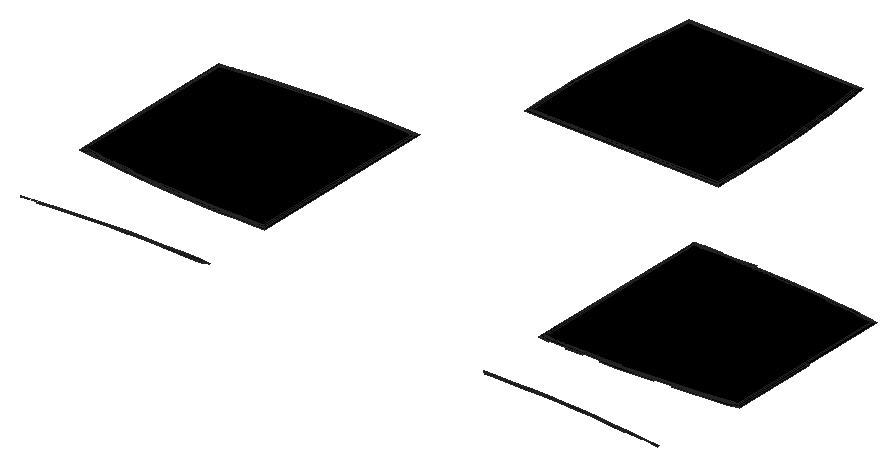
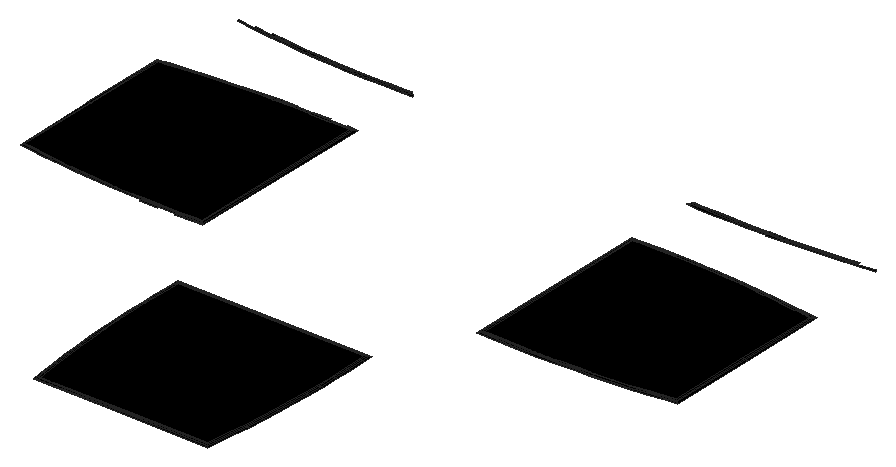
# SketchUp Ruby script. Lengths in inches.
U = 1.inch
M = Sketchup.active_model
def pt(a) = Geom::Point3d.new(a.map { |v| v * U })
def face(e, loops, mat)
  f = e.add_face(loops[0].map { |a| pt(a) })
  loops[1..].each { |l| e.add_face(l.map { |a| pt(a) }).erase! }
  f.material = f.back_material = mat if mat
  f
end
# faces: each face lists its corners as indices into pts; further lists are holes
def faces(e, pts, list, mat = nil) = list.each { |f| face(e, (f[0].is_a?(Array) ? f : [f]).map { |l| l.map { |i| pts[i] } }, mat) }
# xy, xz, yz: faces in a plane at the given z, y or x. An outline is a flat list of corners, or four numbers for a rectangle; further outlines are holes
def ring(l) = l.size == 4 ? [[l[0], l[1]], [l[2], l[1]], [l[2], l[3]], [l[0], l[3]]] : l.each_slice(2).to_a
def flat(e, list, mat, &to3) = list.each { |f| face(e, (f[0].is_a?(Array) ? f : [f]).map { |l| ring(l).map { |u, v| to3.(u, v) } }, mat) }
def xy(e, z, list, mat = nil) = flat(e, list, mat) { |x, y| [x, y, z] }
def xz(e, y, list, mat = nil) = flat(e, list, mat) { |x, z| [x, y, z] }
def yz(e, x, list, mat = nil) = flat(e, list, mat) { |y, z| [x, y, z] }
def lines(e, pts, list) = list.each { |a, b| e.add_line(pt(pts[a]), pt(pts[b])) }
# prism: a flat outline (further loops are holes) pulled along v
def prism(e, loops, v, mat = nil)
  f = face(e, loops, mat); d = Geom::Vector3d.new(v.map { |x| x * U })
  f.pushpull(f.normal.samedirection?(d) ? d.length : -d.length)
end
def box(e, o, s, mat = nil) = prism(e, [[o, [o[0] + s[0], o[1], o[2]], [o[0] + s[0], o[1] + s[1], o[2]], [o[0], o[1] + s[1], o[2]]]], [0, 0, s[2]], mat)
def at(x, y, z, deg = 0) = Geom::Transformation.translation(pt([x, y, z])) * Geom::Transformation.rotation(ORIGIN, Z_AXIS, deg.degrees)
def axes(o, x, y, z) = Geom::Transformation.new([*x, 0, *y, 0, *z, 0, *pt(o).to_a, 1])
def part(name) = M.definitions.add(name)
# library, detail: a bought-in or finely detailed component or shape, given as its bounding box
def library(name, o, s) = part(name).tap { |d| box(d.entities, o, s) }
def detail(e, o, s) = box(e.add_group.entities, o, s)
def put(e, d, t, mat = nil) = e.add_instance(d, t).tap { |i| i.material = mat if mat }
def group(e, t, mat = nil) = e.add_group.tap { |g| g.transformation = t; g.material = mat if mat }.entities
root = M.entities
M.materials.add("[Color M09]").color = [0, 0, 0]
xy(root,29.97,[[96.41,139.98,98.1,140,99.78,140.04,100.4,140.0625,100.4,158.33,99.78,158.35,98.1,158.39,96.41,158.41,94.72,158.39,93.04,158.35,93.02,158.35,91.35,158.28,89.66,158.18,87.98,158.06,86.3,157.9,84.62,157.72,82.94,157.51,82.23,157.41,82.23,140.98,82.94,140.88,84.62,140.67,86.3,140.49,87.98,140.33,89.66,140.21,91.35,140.11,93.02,140.04,93.04,140.04,94.72,140],[132.31,139.98,134,140,135.68,140.04,135.7,140.04,137.375,140.11,139.0625,140.21,140.75,140.33,142.43,140.49,144.1,140.67,145.78,140.88,146.49,140.98,146.49,157.41,145.78,157.51,144.1,157.72,142.43,157.9,140.75,158.06,139.0625,158.18,137.375,158.28,135.7,158.35,135.68,158.35,134,158.39,132.31,158.41,130.625,158.39,128.9375,158.35,128.32,158.33,128.32,140.0625,128.9375,140.04,130.625,140],[105.23,167.19,123.49,167.19,123.52,167.8125,123.56,169.5,123.57,171.1875,123.56,172.875,123.52,174.55,123.52,174.57,123.45,176.25,123.35,177.93,123.22,179.62,123.07,181.3,122.89,182.98,122.68,184.65,122.58,185.37,106.15,185.37,106.05,184.65,105.84,182.98,105.65,181.3,105.5,179.62,105.375,177.93,105.28,176.25,105.21,174.57,105.21,174.55,105.16,172.875,105.15,171.1875,105.16,169.5,105.21,167.8125]],"[Color M09]")
p = [[84.59,132.1,29.93],[84.57,132.24,29.89],[82.89,132.03,29.89],[82.91,131.89,29.93],[144.15,132.24,29.89],[144.14,132.1,29.93],
  [145.82,131.89,29.93],[145.84,132.03,29.89],[86.28,132.14,29.96],[86.27,132.28,29.93],[84.6,131.96,29.96],[142.46,132.28,29.93],
  [142.44,132.14,29.96],[144.12,131.96,29.96],[86.25,132.42,29.89],[87.97,132.3,29.96],[87.95,132.44,29.93],[140.77,132.44,29.93],
  [140.76,132.3,29.96],[142.47,132.42,29.89],[87.94,132.58,29.89],[89.65,132.42,29.96],[89.64,132.57,29.93],[139.08,132.57,29.93],
  [139.07,132.42,29.96],[140.78,132.58,29.89],[89.63,132.71,29.89],[91.34,132.52,29.96],[91.33,132.66,29.93],[137.39,132.66,29.93],
  [137.38,132.52,29.96],[139.09,132.71,29.89],[93.02,132.74,29.93],[93.02,132.59,29.96],[135.71,132.74,29.93],[135.7,132.59,29.96],
  [91.33,132.8,29.89],[93.04,132.59,29.96],[93.03,132.74,29.93],[94.72,132.78,29.93],[94.72,132.63,29.96],[96.41,132.79,29.93],
  [96.41,132.65,29.96],[98.1,132.78,29.93],[98.1,132.63,29.96],[99.79,132.74,29.93],[99.79,132.59,29.96],[100.69,132.7,29.93],
  [100.55,132.56,29.96],[128.93,132.74,29.93],[128.93,132.59,29.96],[128.18,132.56,29.96],[128.03,132.7,29.93],[130.62,132.78,29.93],
  [130.625,132.63,29.96],[132.31,132.79,29.93],[132.31,132.65,29.96],[134.01,132.78,29.93],[134.01,132.63,29.96],[135.69,132.74,29.93],
  [135.6875,132.59,29.96],[137.4,132.8,29.89],[93.01,132.875,29.89],[93.02,132.875,29.89],[94.71,132.92,29.89],[98.1,132.92,29.89],
  [99.8,132.875,29.89],[100.83,132.83,29.89],[128.92,132.875,29.89],[127.89,132.83,29.89],[130.62,132.92,29.89],[134.01,132.92,29.89],
  [135.7,132.875,29.89],[135.71,132.875,29.89],[96.41,132.93,29.89],[132.31,132.93,29.89],[91.33,139.68,29.89],[93.01,139.61,29.89],
  [93.02,139.75,29.93],[91.33,139.82,29.93],[94.71,139.57,29.89],[93.02,139.61,29.89],[93.03,139.75,29.93],[94.72,139.7,29.93],
  [96.41,139.69,29.93],[96.41,139.55,29.89],[98.1,139.7,29.93],[98.1,139.56,29.89],[99.79,139.75,29.93],[99.8,139.61,29.89],
  [100.69,139.78,29.93],[100.83,139.65,29.89],[100.69,158.6,29.93],[100.83,158.74,29.89],[128.93,139.75,29.93],[128.92,139.61,29.89],
  [127.89,139.65,29.89],[128.03,139.78,29.93],[127.89,158.74,29.89],[128.03,158.6,29.93],[132.31,139.69,29.93],[132.31,139.55,29.89],
  [130.62,139.56,29.89],[130.62,139.7,29.93],[135.7,139.61,29.89],[134.01,139.57,29.89],[134.01,139.7,29.93],[135.69,139.75,29.93],
  [135.71,139.61,29.89],[137.4,139.68,29.89],[137.39,139.82,29.93],[135.71,139.75,29.93],[89.64,139.92,29.93],[89.63,139.78,29.89],
  [93.02,139.89,29.96],[91.34,139.96,29.96],[93.04,139.89,29.96],[94.72,139.85,29.96],[96.41,139.83,29.96],[98.1,139.85,29.96],
  [99.79,139.89,29.96],[100.55,139.92,29.96],[128.93,139.89,29.96],[128.18,139.92,29.96],[130.625,139.85,29.96],[132.31,139.83,29.96],
  [134.01,139.85,29.96],[135.6875,139.89,29.96],[135.7,139.89,29.96],[137.38,139.96,29.96],[139.09,139.78,29.89],[139.08,139.92,29.93],
  [87.95,140.04,29.93],[87.94,139.9,29.89],[89.65,140.06,29.96],[100.55,158.47,29.96],[128.18,158.47,29.96],[139.07,140.06,29.96],
  [86.27,140.2,29.93],[86.25,140.06,29.89],[87.97,140.1875,29.96],[140.77,140.04,29.93],[140.76,140.1875,29.96],[140.78,139.9,29.89],
  [142.47,140.06,29.89],[142.46,140.2,29.93],[86.28,140.34,29.96],[142.44,140.34,29.96],[84.59,140.38,29.93],[84.57,140.24,29.89],
  [144.15,140.24,29.89],[144.14,140.38,29.93],[82.91,140.59,29.93],[82.89,140.45,29.89],[84.6,140.52,29.96],[144.12,140.52,29.96],
  [145.84,140.45,29.89],[145.82,140.59,29.93],[82.92,140.73,29.96],[145.8,140.73,29.96],[81.9375,140.73,29.93],[81.8,140.61,29.89],
  [146.92,140.61,29.89],[146.78,140.73,29.93],[81.9375,149.19,29.93],[81.8,149.19,29.89],[82.08,140.85,29.96],[146.64,140.85,29.96],
  [146.92,149.19,29.89],[146.78,149.19,29.93],[82.08,149.19,29.96],[146.64,149.19,29.96],[81.9375,157.66,29.93],[81.8,157.78,29.89],
  [82.08,157.53,29.96],[146.78,157.66,29.93],[146.64,157.53,29.96],[82.92,157.65,29.96],[82.91,157.8,29.93],[145.82,157.8,29.93],
  [145.8,157.65,29.96],[82.89,157.9375,29.89],[84.6,157.86,29.96],[84.59,158.01,29.93],[144.14,158.01,29.93],[144.12,157.86,29.96],
  [84.57,158.15,29.89],[86.28,158.05,29.96],[86.27,158.19,29.93],[142.46,158.19,29.93],[142.44,158.05,29.96],[86.25,158.33,29.89],
  [87.97,158.2,29.96],[87.95,158.35,29.93],[140.77,158.35,29.93],[140.76,158.2,29.96],[87.94,158.48,29.89],[89.65,158.33,29.96],
  [89.64,158.47,29.93],[139.08,158.47,29.93],[139.07,158.33,29.96],[89.63,158.61,29.89],[91.34,158.43,29.96],[91.33,158.57,29.93],
  [137.39,158.57,29.93],[137.38,158.43,29.96],[93.02,158.64,29.93],[93.02,158.5,29.96],[135.71,158.64,29.93],[135.7,158.5,29.96],
  [91.33,158.71,29.89],[93.04,158.5,29.96],[93.03,158.64,29.93],[94.72,158.68,29.93],[94.72,158.54,29.96],[96.41,158.7,29.93],
  [96.41,158.55,29.96],[98.1,158.68,29.93],[98.1,158.54,29.96],[99.79,158.64,29.93],[99.79,158.5,29.96],[128.93,158.64,29.93],
  [128.93,158.5,29.96],[130.62,158.68,29.93],[130.625,158.54,29.96],[132.31,158.7,29.93],[132.31,158.55,29.96],[134.01,158.68,29.93],
  [134.01,158.54,29.96],[135.69,158.64,29.93],[135.6875,158.5,29.96],[93.01,158.78,29.89],[93.02,158.78,29.89],[94.71,158.82,29.89],
  [98.1,158.82,29.89],[99.8,158.78,29.89],[128.92,158.78,29.89],[130.62,158.82,29.89],[96.41,158.84,29.89],[134.01,158.82,29.89],
  [132.31,158.84,29.89],[123.77,166.9,29.93],[123.91,166.76,29.89],[104.82,166.76,29.89],[104.95,166.9,29.93],[104.77,167.8,29.89],
  [104.91,167.8,29.93],[123.81,167.8,29.93],[123.95,167.8,29.89],[105.06,167.81,29.96],[105.09,167.05,29.96],[123.63,167.05,29.96],
  [123.67,167.81,29.96],[104.73,169.49,29.89],[104.87,169.49,29.93],[105.02,169.5,29.96],[123.71,169.5,29.96],[123.85,169.49,29.93],
  [123.99,169.49,29.89],[104.72,171.1875,29.89],[104.86,171.1875,29.93],[105,171.1875,29.96],[123.72,171.1875,29.96],[123.87,171.1875,29.93],
  [124,171.1875,29.89],[104.73,172.88,29.89],[104.87,172.88,29.93],[105.02,172.88,29.96],[123.71,172.88,29.96],[123.85,172.88,29.93],
  [123.99,172.88,29.89],[104.78,174.57,29.89],[104.91,174.57,29.93],[105.06,174.56,29.96],[123.81,174.57,29.93],[123.67,174.56,29.96],
  [123.95,174.57,29.89],[104.91,174.58,29.93],[104.78,174.58,29.89],[104.85,176.27,29.89],[104.99,176.26,29.93],[105.06,174.58,29.96],
  [105.13,176.26,29.96],[123.81,174.58,29.93],[123.74,176.26,29.93],[123.59,176.26,29.96],[123.66,174.58,29.96],[123.95,174.58,29.89],
  [123.88,176.27,29.89],[105.08,177.95,29.93],[104.94,177.96,29.89],[105.23,177.94,29.96],[123.64,177.95,29.93],[123.5,177.94,29.96],
  [123.78,177.96,29.89],[105.35,179.63,29.96],[105.21,179.64,29.93],[123.51,179.64,29.93],[123.37,179.63,29.96],[105.07,179.65,29.89],
  [123.65,179.65,29.89],[105.37,181.33,29.93],[105.23,181.34,29.89],[105.51,181.3125,29.96],[123.36,181.33,29.93],[123.21,181.3125,29.96],
  [123.5,181.34,29.89],[105.55,183.01,29.93],[105.41,183.03,29.89],[105.69,182.99,29.96],[123.18,183.01,29.93],[123.03,182.99,29.96],
  [123.3125,183.03,29.89],[105.76,184.69,29.93],[105.62,184.71,29.89],[105.9,184.67,29.96],[122.97,184.69,29.93],[122.82,184.67,29.96],
  [123.1,184.71,29.89],[105.9,185.66,29.93],[105.77,185.8,29.89],[106.02,185.51,29.96],[122.83,185.66,29.93],[122.7,185.51,29.96],
  [122.95,185.8,29.89],[114.36,185.51,29.96],[114.36,185.66,29.93],[114.36,185.8,29.89],[86.3,132,29.97],[84.62,131.8125,29.97],
  [87.98,132.15,29.97],[140.75,132.15,29.97],[142.43,132,29.97],[89.66,132.28,29.97],[139.0625,132.28,29.97],[91.35,132.375,29.97],
  [137.375,132.375,29.97],[93.02,132.44,29.97],[93.04,132.44,29.97],[94.72,132.49,29.97],[98.1,132.49,29.97],[99.78,132.44,29.97],
  [100.4,132.42,29.97],[128.9375,132.44,29.97],[128.32,132.42,29.97],[130.625,132.49,29.97],[135.68,132.44,29.97],[134,132.49,29.97],
  [135.7,132.44,29.97],[96.41,132.5,29.97],[132.31,132.5,29.97],[93.04,140.04,29.97],[94.72,140,29.97],[96.41,139.98,29.97],
  [98.1,140,29.97],[99.78,140.04,29.97],[130.625,140,29.97],[128.9375,140.04,29.97],[132.31,139.98,29.97],[134,140,29.97],
  [135.68,140.04,29.97],[93.02,140.04,29.97],[91.35,140.11,29.97],[100.4,140.0625,29.97],[100.4,158.33,29.97],[128.32,140.0625,29.97],
  [128.32,158.33,29.97],[135.7,140.04,29.97],[137.375,140.11,29.97],[89.66,140.21,29.97],[139.0625,140.21,29.97],[87.98,140.33,29.97],
  [140.75,140.33,29.97],[86.3,140.49,29.97],[142.43,140.49,29.97],[84.62,140.67,29.97],[144.1,140.67,29.97],[82.94,140.88,29.97],
  [145.78,140.88,29.97],[82.23,140.98,29.97],[146.49,140.98,29.97],[82.23,149.19,29.97],[146.49,149.19,29.97],[82.23,157.41,29.97],
  [146.49,157.41,29.97],[82.94,157.51,29.97],[145.78,157.51,29.97],[84.62,157.72,29.97],[144.1,157.72,29.97],[86.3,157.9,29.97],
  [142.43,157.9,29.97],[87.98,158.06,29.97],[140.75,158.06,29.97],[89.66,158.18,29.97],[139.0625,158.18,29.97],[91.35,158.28,29.97],
  [137.375,158.28,29.97],[93.02,158.35,29.97],[93.04,158.35,29.97],[99.78,158.35,29.97],[128.9375,158.35,29.97],[135.7,158.35,29.97],
  [135.68,158.35,29.97],[94.72,158.39,29.97],[96.41,158.41,29.97],[98.1,158.39,29.97],[130.625,158.39,29.97],[132.31,158.41,29.97],
  [134,158.39,29.97],[123.49,167.19,29.97],[105.23,167.19,29.97],[105.21,167.8125,29.97],[123.52,167.8125,29.97],[105.16,169.5,29.97],
  [123.56,169.5,29.97],[105.15,171.1875,29.97],[123.57,171.1875,29.97],[105.16,172.875,29.97],[123.56,172.875,29.97],[105.21,174.55,29.97],
  [123.52,174.55,29.97],[105.21,174.57,29.97],[105.28,176.25,29.97],[123.45,176.25,29.97],[123.52,174.57,29.97],[105.375,177.93,29.97],
  [123.35,177.93,29.97],[105.5,179.62,29.97],[123.22,179.62,29.97],[105.65,181.3,29.97],[123.07,181.3,29.97],[105.84,182.98,29.97],
  [122.89,182.98,29.97],[106.05,184.65,29.97],[122.68,184.65,29.97],[106.15,185.37,29.97],[122.58,185.37,29.97],[114.36,185.37,29.97]]
faces(root,p,[[0,1,2,3],[4,5,6,7],[8,9,0,10],[11,12,13,5],[9,14,1,0],[15,16,9,8],[17,18,12,11],[19,11,5,4],
  [16,20,14,9],[21,22,16,15],[23,24,18,17],[25,17,11,19],[22,26,20,16],[27,28,22,21],[29,30,24,23],[31,23,17,25],
  [32,28,27,33],[29,34,35,30],[28,36,26,22],[37,33,32,38],[38,39,40,37],[40,39,41,42],[42,41,43,44],[44,43,45,46],
  [46,45,47,48],[49,50,51,52],[53,54,50,49],[55,56,54,53],[57,58,56,55],[57,59,60,58],[60,35,34,59],[61,29,23,31],
  [62,36,28,32],[38,32,62,63],[63,64,39,38],[43,65,66,45],[45,66,67,47],[68,49,52,69],[70,53,49,68],[71,72,59,57],
  [61,73,34,29],[59,34,73,72],[39,64,74,41],[41,74,65,43],[75,55,53,70],[71,57,55,75],[76,77,78,79],[80,81,82,83],
  [82,78,77,81],[80,83,84,85],[85,84,86,87],[87,86,88,89],[89,88,90,91],[92,93,91,90],[94,95,96,97],[97,96,98,99],
  [100,101,102,103],[104,105,106,107],[108,109,110,111],[76,79,112,113],[79,78,114,115],[83,82,116,117],[116,114,78,82],[83,117,118,84],
  [84,118,119,86],[86,119,120,88],[88,120,121,90],[122,94,97,123],[124,103,94,122],[125,100,103,124],[126,106,100,125],[107,106,126,127],
  [127,128,111,107],[111,110,129,128],[110,109,130,131],[113,112,132,133],[79,115,134,112],[135,92,90,121],[123,97,99,136],[129,110,131,137],
  [133,132,138,139],[112,134,140,132],[137,131,141,142],[141,143,144,145],[132,140,146,138],[142,141,145,147],[139,138,148,149],[145,144,150,151],
  [149,148,152,153],[138,146,154,148],[147,145,151,155],[151,150,156,157],[148,154,158,152],[155,151,157,159],[153,152,160,161],[157,156,162,163],
  [161,160,164,165],[152,158,166,160],[159,157,163,167],[163,162,168,169],[160,166,170,164],[167,163,169,171],[172,173,165,164],[174,172,164,170],
  [175,176,171,169],[177,178,172,174],[179,180,176,175],[178,181,173,172],[182,183,178,177],[184,185,180,179],[183,186,181,178],[187,188,183,182],
  [189,190,185,184],[188,191,186,183],[192,193,188,187],[194,195,190,189],[193,196,191,188],[197,198,193,192],[199,200,195,194],[198,201,196,193],
  [202,203,198,197],[204,205,200,199],[206,203,202,207],[204,208,209,205],[203,210,201,198],[211,207,206,212],[212,213,214,211],[214,213,215,216],
  [216,215,217,218],[218,217,219,220],[220,219,92,135],[221,222,136,99],[223,224,222,221],[225,226,224,223],[227,228,226,225],[227,229,230,228],
  [230,209,208,229],[231,210,203,206],[212,206,231,232],[232,233,213,212],[217,234,235,219],[219,235,93,92],[236,221,99,98],[237,223,221,236],
  [213,233,238,215],[215,238,234,217],[239,227,225,240],[241,242,243,244],[245,246,244,243],[247,248,242,241],[246,249,250,244],[251,241,244,250],
  [252,247,241,251],[253,254,246,245],[254,255,249,246],[256,257,247,252],[257,258,248,247],[259,260,254,253],[260,261,255,254],[262,263,257,256],
  [263,264,258,257],[265,266,260,259],[266,267,261,260],[268,269,263,262],[269,270,264,263],[265,271,272,266],[266,272,273,267],[274,269,268,275],
  [276,270,269,274],[272,277,278,271],[279,278,277,280],[273,281,277,272],[280,277,281,282],[283,284,285,286],[275,286,283,274],[287,288,284,283],
  [274,283,287,276],[279,280,289,290],[280,282,291,289],[285,284,292,293],[284,288,294,292],[289,291,295,296],[293,292,297,298],[290,289,296,299],
  [292,294,300,297],[299,296,301,302],[296,295,303,301],[298,297,304,305],[297,300,306,304],[302,301,307,308],[301,303,309,307],[305,304,310,311],
  [304,306,312,310],[308,307,313,314],[307,309,315,313],[311,310,316,317],[310,312,318,316],[314,313,319,320],[313,315,321,319],[317,316,322,323],
  [316,318,324,322],[319,321,325,326],[323,322,326,325],[320,319,326,327],[322,324,327,326],[328,8,10,329],[330,15,8,328],[18,331,332,12],
  [333,21,15,330],[24,334,331,18],[335,27,21,333],[30,336,334,24],[33,27,335,337],[338,337,33,37],[37,40,339,338],[340,44,46,341],
  [341,46,48,342],[50,343,344,51],[54,345,343,50],[58,60,346,347],[30,35,348,336],[346,348,35,60],[339,40,42,349],[349,42,44,340],
  [56,350,345,54],[58,347,350,56],[117,116,351,352],[117,352,353,118],[118,353,354,119],[119,354,355,120],[356,124,122,357],[358,125,124,356],
  [359,126,125,358],[127,126,359,360],[115,114,361,362],[351,361,114,116],[120,355,363,121],[364,135,121,363],[357,122,123,365],[365,123,136,366],
  [360,367,128,127],[128,129,368,367],[115,362,369,134],[368,129,137,370],[134,369,371,140],[370,137,142,372],[140,371,373,146],[372,142,147,374],
  [146,373,375,154],[374,147,155,376],[154,375,377,158],[376,155,159,378],[158,377,379,166],[378,159,167,380],[166,379,381,170],[380,167,171,382],
  [383,174,170,381],[176,384,382,171],[385,177,174,383],[180,386,384,176],[387,182,177,385],[185,388,386,180],[389,187,182,387],[190,390,388,185],
  [391,192,187,389],[195,392,390,190],[393,197,192,391],[200,394,392,195],[395,202,197,393],[205,396,394,200],[207,202,395,397],[398,397,207,211],
  [399,220,135,364],[222,400,366,136],[205,209,401,396],[402,401,209,230],[211,214,403,398],[403,214,216,404],[404,216,218,405],[405,218,220,399],
  [224,406,400,222],[226,407,406,224],[228,408,407,226],[228,230,402,408],[409,251,250,410],[249,411,410,250],[412,252,251,409],[255,413,411,249],
  [414,256,252,412],[261,415,413,255],[416,262,256,414],[267,417,415,261],[418,268,262,416],[267,273,419,417],[275,268,418,420],[419,421,281,273],
  [282,281,421,422],[286,285,423,424],[420,424,286,275],[282,422,425,291],[423,285,293,426],[291,425,427,295],[426,293,298,428],[295,427,429,303],
  [428,298,305,430],[303,429,431,309],[430,305,311,432],[309,431,433,315],[432,311,317,434],[315,433,435,321],[434,317,323,436],[321,435,437,325],
  [436,323,325,437]],"[Color M09]")
